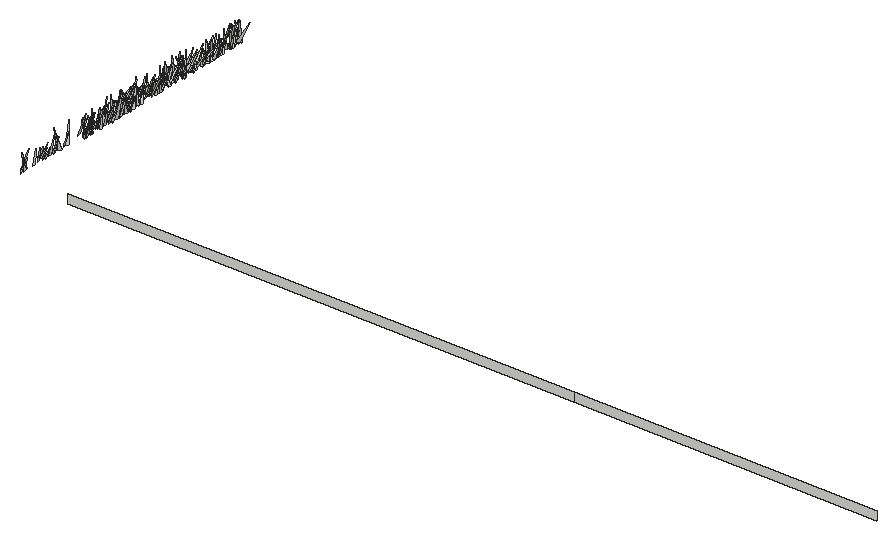
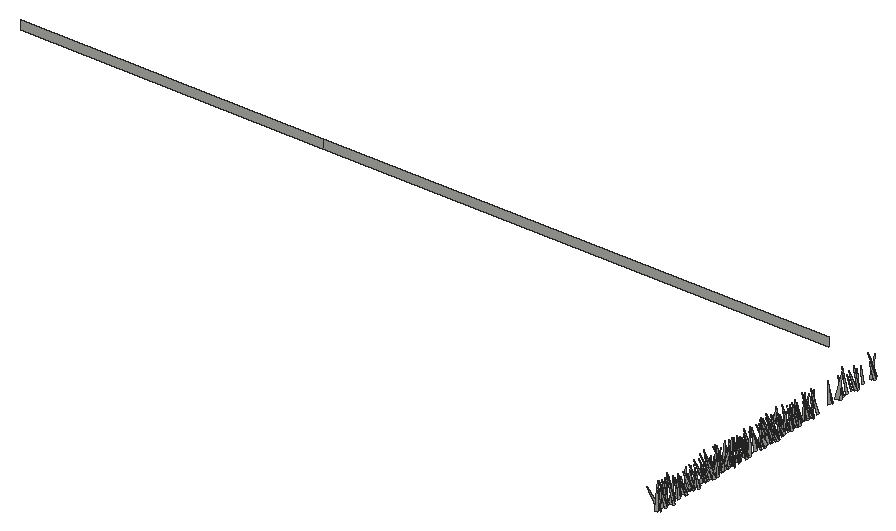
# SketchUp Ruby script. Lengths in inches.
U = 1.inch
M = Sketchup.active_model
def pt(a) = Geom::Point3d.new(a.map { |v| v * U })
def face(e, loops, mat)
  f = e.add_face(loops[0].map { |a| pt(a) })
  loops[1..].each { |l| e.add_face(l.map { |a| pt(a) }).erase! }
  f.material = f.back_material = mat if mat
  f
end
# faces: each face lists its corners as indices into pts; further lists are holes
def faces(e, pts, list, mat = nil) = list.each { |f| face(e, (f[0].is_a?(Array) ? f : [f]).map { |l| l.map { |i| pts[i] } }, mat) }
# xy, xz, yz: faces in a plane at the given z, y or x. An outline is a flat list of corners, or four numbers for a rectangle; further outlines are holes
def ring(l) = l.size == 4 ? [[l[0], l[1]], [l[2], l[1]], [l[2], l[3]], [l[0], l[3]]] : l.each_slice(2).to_a
def flat(e, list, mat, &to3) = list.each { |f| face(e, (f[0].is_a?(Array) ? f : [f]).map { |l| ring(l).map { |u, v| to3.(u, v) } }, mat) }
def xy(e, z, list, mat = nil) = flat(e, list, mat) { |x, y| [x, y, z] }
def xz(e, y, list, mat = nil) = flat(e, list, mat) { |x, z| [x, y, z] }
def yz(e, x, list, mat = nil) = flat(e, list, mat) { |y, z| [x, y, z] }
def lines(e, pts, list) = list.each { |a, b| e.add_line(pt(pts[a]), pt(pts[b])) }
# prism: a flat outline (further loops are holes) pulled along v
def prism(e, loops, v, mat = nil)
  f = face(e, loops, mat); d = Geom::Vector3d.new(v.map { |x| x * U })
  f.pushpull(f.normal.samedirection?(d) ? d.length : -d.length)
end
def box(e, o, s, mat = nil) = prism(e, [[o, [o[0] + s[0], o[1], o[2]], [o[0] + s[0], o[1] + s[1], o[2]], [o[0], o[1] + s[1], o[2]]]], [0, 0, s[2]], mat)
def at(x, y, z, deg = 0) = Geom::Transformation.translation(pt([x, y, z])) * Geom::Transformation.rotation(ORIGIN, Z_AXIS, deg.degrees)
def axes(o, x, y, z) = Geom::Transformation.new([*x, 0, *y, 0, *z, 0, *pt(o).to_a, 1])
def part(name) = M.definitions.add(name)
# library, detail: a bought-in or finely detailed component or shape, given as its bounding box
def library(name, o, s) = part(name).tap { |d| box(d.entities, o, s) }
def detail(e, o, s) = box(e.add_group.entities, o, s)
def put(e, d, t, mat = nil) = e.add_instance(d, t).tap { |i| i.material = mat if mat }
def group(e, t, mat = nil) = e.add_group.tap { |g| g.transformation = t; g.material = mat if mat }.entities
root = M.entities
c1 = part("fur_instance\#9")
p = [[0.8125,0,1.79],[0.67,-0.02,1.48],[0,-0.11,0],[0,0.11,0]]
faces(c1.entities,p,[[0,1,2,3]])
xz(root,5.77,[[196.6875,-27.625,525.63,-21.625],[525.63,-27.625,722.32,-21.625]])
put(root,c1,axes([157.51,131.72,-27.1],[2.91311,4.64162,1.0633],[4.76072,-2.81168,-0.76908],[0.10392,-1.30816,5.4258]))
put(root,c1,axes([159.54,140.72,-28.22],[-2.17535,-3.01047,0.60266],[-3.06621,2.16789,-0.23847],[0.15643,0.62897,3.70651]))
put(root,c1,axes([157.26,67.54,-28.22],[4.29125,3.34973,1.68987],[3.74545,-3.97458,-1.63261],[-0.21889,-2.33948,5.19327]))
put(root,c1,axes([160.47,87.49,-28.22],[-7.01031,-0.43579,1.43561],[-0.72042,6.99511,-1.39453],[1.31601,1.50792,6.88401]))
put(root,c1,axes([158.58,119.34,-28.22],[3.7026,-0.58317,1.91769],[-1.4169,-3.61072,1.63767],[-1.41775,2.08554,3.37155]))
put(root,c1,axes([156.99,160.79,-28.22],[0.56131,-6.10589,2.64479],[-6.41112,0.21442,1.85565],[1.78167,2.69518,5.8441]))
put(root,c1,axes([157.16,88.07,-27.1],[4.10425,1.09153,0.3293],[1.14011,-3.92312,-1.20584],[0.00571,-1.24998,4.07214]))
put(root,c1,axes([157.71,140.53,-27.1],[-1.05079,-7.8114,1.55453],[-7.7743,1.34665,1.51176],[1.73053,1.30661,7.73542]))
put(root,c1,axes([160.65,168.01,-28.22],[-4.27711,1.68369,0.0136],[1.68167,4.26988,0.26227],[-0.08344,-0.24902,4.58909]))
put(root,c1,axes([159.34,137.68,-28.22],[-4.78026,1.17069,2.19317],[1.89155,4.79719,1.56216],[1.61324,-2.15588,4.66702]))
put(root,c1,axes([156.68,18.28,-27.1],[2.75762,-4.13306,0.47465],[-3.98702,-2.46295,1.71739],[1.18791,1.32801,4.66232]))
put(root,c1,axes([156.68,188.21,-27.1],[2.75762,-4.13306,0.47465],[-3.98702,-2.46295,1.71739],[1.18791,1.32801,4.66232]))
put(root,c1,axes([158.6,80.15,-28.22],[-2.21972,3.26489,1.22418],[3.2229,2.47495,-0.75684],[1.3308,-0.54808,3.87477]))
put(root,c1,axes([159.18,164.24,-28.22],[-4.17455,0.44699,1.70239],[0.80041,4.38471,0.81146],[1.56757,-1.04848,4.11925]))
put(root,c1,axes([158.22,175.8125,-28.22],[4.13906,-0.88394,1.08396],[-0.87234,-4.27812,-0.15771],[-1.09332,0.06702,4.22946]))
put(root,c1,axes([159.26,127.18,-28.22],[6.19428,-1.57461,3.33029],[-1.87234,-6.95675,0.19327],[-3.17247,1.03131,6.38836]))
put(root,c1,axes([159.34,169.26,-28.22],[3.93388,5.26717,1.14139],[4.90502,-4.08461,1.94372],[-2.23307,0.30691,6.28017]))
put(root,c1,axes([157.5,170.05,-28.22],[4.34496,-0.35551,0.43941],[-0.4633,-4.19131,1.19014],[-0.32376,1.22666,4.19388]))
put(root,c1,axes([156.92,131.9,-28.22],[6.72288,3.05704,0.61475],[3.02645,-6.7488,0.46346],[-0.75102,0.16938,7.37074]))
put(root,c1,axes([157.94,132.77,-27.1],[-1.4348,-7.0433,2.45033],[-7.23254,1.92235,1.29061],[1.81726,2.08982,7.07114]))
put(root,c1,axes([159.1875,81.03,-28.22],[5.31201,5.41879,2.20999],[5.24419,-5.73235,1.45032],[-2.59727,-0.49162,7.44831]))
put(root,c1,axes([158.99,52.21,-27.1],[5.64429,-3.09602,3.33103],[-3.78051,-6.14532,0.69416],[-2.52761,2.27789,6.40012]))
put(root,c1,axes([159.05,102.86,-28.22],[2.70237,-4.42657,2.31196],[-4.83243,-2.98105,-0.05917],[-1.25989,1.93941,5.18593]))
put(root,c1,axes([158.375,149.63,-27.1],[-2.24137,-6.8028,0.2078],[-6.58087,2.22202,1.76064],[1.73594,-0.35988,6.94277]))
put(root,c1,axes([157.875,84.56,-28.22],[5.31281,-2.73186,1.51927],[-2.91837,-5.40827,0.48055],[-1.11999,1.13346,5.95467]))
put(root,c1,axes([160.2,108.16,-28.22],[-0.94907,-6.99906,3.73248],[-7.88487,0.42284,-1.21201],[-0.8643,3.82797,6.95835]))
put(root,c1,axes([157.1,33.07,-27.1],[5.55155,-0.72144,0.45458],[-0.77671,-5.51397,0.73462],[-0.35191,0.78896,5.54982]))
put(root,c1,axes([158.86,147.7,-28.22],[4.52461,-6.7861,0.00105],[-6.53347,-4.35651,-2.20405],[-1.83437,-1.22185,7.85273]))
put(root,c1,axes([158.53,76.12,-27.1],[0.17579,4.7582,1.26729],[4.89735,-0.03702,-0.54033],[0.51227,-1.27889,4.73069]))
put(root,c1,axes([156.77,181.63,-28.22],[-0.81294,-7.33898,4.00432],[-7.82592,2.08335,2.22952],[2.94113,3.51498,7.03923]))
put(root,c1,axes([158.62,108.45,-27.1],[3.88995,3.95886,0.07672],[3.75671,-3.72392,1.68217],[-1.25122,1.12695,5.2891]))
put(root,c1,axes([160.78,101.25,-28.22],[-1.75901,-6.72397,0.92553],[-6.70142,1.56883,-1.33876],[-1.07676,1.22044,6.82009]))
put(root,c1,axes([158.23,118.83,-28.22],[6.94101,-3.43299,1.84422],[-3.2352,-7.17632,-1.18245],[-2.17258,-0.28153,7.65277]))
put(root,c1,axes([159.31,89.31,-28.22],[-2.09366,4.25191,0.8072],[4.26644,2.17826,-0.40798],[0.72654,-0.53866,4.72184]))
put(root,c1,axes([157.43,45.27,-27.1],[2.80299,-5.03768,0.10257],[-5.00094,-2.76705,0.76127],[0.6159,0.45904,5.71449]))
put(root,c1,axes([160.36,93.08,-28.22],[-2.25031,-4.2676,0.76277],[-4.32128,2.13921,-0.77999],[-0.34742,1.03417,4.76108]))
put(root,c1,axes([158.22,143.05,-27.1],[-5.21121,-4.35385,3.58957],[-4.50193,6.15376,0.92827],[3.40202,1.4741,6.72689]))
put(root,c1,axes([160.66,133.85,-28.22],[-4.51725,1.3418,0.80765],[1.52463,4.33149,1.33117],[0.35811,-1.51528,4.52039]))
put(root,c1,axes([160.09,91.41,-28.22],[0.93593,4.40998,1.37185],[4.37962,-1.29175,1.16453],[-1.46587,-1.0437,4.3552]))
put(root,c1,axes([158.34,190.83,-28.22],[-3.30417,-4.76212,3.2823],[-5.25525,4.05058,0.5865],[2.41528,2.29867,5.7664]))
put(root,c1,axes([156.31,97,-27.1],[3.48936,7.09192,0.65775],[6.9322,-3.21357,-2.12629],[1.63479,-1.51038,7.61247]))
put(root,c1,axes([156.77,99.2,-27.1],[3.72746,5.46093,0.78491],[5.42353,-3.45332,-1.72965],[1.01153,-1.60767,6.38153]))
put(root,c1,axes([159.01,46.18,-27.1],[4.03591,-7.21522,0.98619],[-7.10178,-4.1491,-1.2924],[-1.61145,0.21471,8.16564]))
put(root,c1,axes([156.96,64.22,-27.1],[7.02887,1.41814,0.69885],[1.44367,-7.05544,-0.2028],[-0.64447,-0.3379,7.16763]))
put(root,c1,axes([156.72,97.48,-28.22],[6.03076,-3.95506,0.64167],[-4.00583,-5.92637,1.12057],[0.08689,1.28836,7.12438]))
put(root,c1,axes([158.94,18.03,-27.1],[5.89812,-2.41371,1.85981],[-1.99813,-6.12286,-1.60962],[-2.30052,-0.87028,6.16628]))
put(root,c1,axes([158.94,187.96,-27.1],[5.89812,-2.41371,1.85981],[-1.99813,-6.12286,-1.60962],[-2.30052,-0.87028,6.16628]))
put(root,c1,axes([160.3,144.44,-28.22],[-3.47143,-2.84551,0.09651],[-2.81271,3.45107,0.57956],[0.4415,-0.38766,4.45106]))
put(root,c1,axes([160.62,66.03,-28.22],[-3.27995,-3.84872,1.10692],[-4.00472,3.15616,-0.89264],[0.01123,1.42196,4.97734]))
put(root,c1,axes([159.04,133.15,-27.1],[-0.27729,4.76979,1.49646],[4.98187,0.38774,-0.31274],[0.41383,-1.47171,4.7676]))
put(root,c1,axes([160.15,145.42,-28.22],[-5.81537,-0.03657,1.70774],[-0.23888,6.01751,-0.6846],[1.69135,0.72416,5.77505]))
put(root,c1,axes([158.2,127.17,-28.22],[4.35259,2.65064,0.87547],[2.69973,-4.40951,-0.0717],[-0.70982,-0.51745,5.09567]))
put(root,c1,axes([159.85,106.57,-28.22],[1.43677,3.63281,1.03111],[3.57622,-1.66329,0.8769],[-1.21291,-0.60083,3.80693]))
put(root,c1,axes([158.41,120.52,-27.1],[2.85218,4.71528,1.10181],[4.83661,-2.83604,-0.38317],[-0.23454,-1.14272,5.49745]))
put(root,c1,axes([159.67,152.3,-28.22],[1.56672,2.93333,1.48069],[3.11219,-1.85095,0.37383],[-1.05412,-1.105,3.30444]))
put(root,c1,axes([158.59,152.92,-28.22],[4.55494,-1.38322,1.77977],[-1.90749,-4.50337,1.38185],[-1.20098,1.9065,4.55536]))
put(root,c1,axes([159.9,164.69,-28.22],[-3.4412,6.39637,0.09759],[6.32165,3.41718,-1.06042],[0.97968,0.41743,7.18546]))
put(root,c1,axes([159.03,92.17,-27.1],[-2.22453,-2.28888,1.93607],[-2.6411,2.63697,0.08289],[1.41842,1.32035,3.19071]))
put(root,c1,axes([158.59,100.56,-27.1],[-1.16046,8.00046,0.20395],[7.87345,1.17823,-1.41992],[1.43448,0.00519,7.95851]))
put(root,c1,axes([158.07,30.12,-27.1],[4.83385,-1.43847,0.54232],[-1.36908,-4.84202,-0.64023],[-0.69925,-0.46374,5.00254]))
put(root,c1,axes([158.26,125.71,-28.22],[4.95919,2.18923,1.00137],[2.21006,-5.04934,0.09393],[-0.95452,-0.31696,5.4201]))
put(root,c1,axes([158.61,19.19,-27.1],[4.29129,-1.7599,0.57931],[-1.53313,-4.1935,-1.38278],[-1.04037,-1.07949,4.42723]))
put(root,c1,axes([158.61,189.125,-27.1],[4.29129,-1.7599,0.57931],[-1.53313,-4.1935,-1.38278],[-1.04037,-1.07949,4.42723]))
put(root,c1,axes([160.19,154.14,-28.22],[2.70067,-3.13661,0.88183],[-2.51329,-2.73437,-2.02883],[-2.07348,-0.77102,3.60774]))
put(root,c1,axes([158.07,100.87,-28.22],[5.62974,5.25868,1.12192],[5.27805,-5.71471,0.30107],[-1.02693,-0.54292,7.69786]))
put(root,c1,axes([158.71,70.54,-27.1],[3.49135,-1.63355,1.08284],[-1.80913,-3.53699,0.49727],[-0.7537,0.9229,3.8224]))
put(root,c1,axes([158.75,133.85,-28.22],[-0.66532,-4.77379,0.4836],[-4.67341,0.75535,1.0268],[1.0873,0.32553,4.70929]))
put(root,c1,axes([156.36,111.21,-27.1],[1.31269,5.55847,0.82299],[4.82858,-0.68361,-3.08457],[2.8738,-1.39037,4.80678]))
put(root,c1,axes([157.73,67.33,-28.22],[-0.77489,5.32124,0.74593],[4.8544,1.01638,-2.20776],[2.30365,-0.35187,4.90325]))
put(root,c1,axes([158.58,77.17,-28.22],[6.13024,0.22864,1.74835],[0.20896,-6.37456,0.10097],[-1.75081,0.03976,6.13367]))
put(root,c1,axes([159.04,112.39,-28.22],[-5.57842,3.33095,2.99608],[3.28064,6.29556,-0.89096],[3.05108,-0.67911,6.43585]))
put(root,c1,axes([158.82,181.64,-28.22],[6.05759,-4.04132,1.47541],[-3.82561,-6.22554,-1.34569],[-1.96821,-0.33746,7.15653]))
put(root,c1,axes([158.15,126.125,-28.22],[5.73568,-0.06882,1.05766],[0.01363,-5.81521,-0.45231],[-1.05981,-0.44725,5.71823]))
put(root,c1,axes([156.54,31.98,-27.1],[0.60809,-6.43634,0.77652],[-5.71222,-0.16309,3.1214],[3.06594,0.97271,5.66154]))
put(root,c1,axes([157.8,132.78,-27.1],[7.1612,-0.61813,1.17268],[-0.1707,-6.81898,-2.55193],[-1.31459,-2.48182,6.71956]))
put(root,c1,axes([159.02,25.45,-27.1],[4.44334,-1.86269,1.64457],[-2.02269,-4.66849,0.17731],[-1.44323,0.80817,4.81471]))
put(root,c1,axes([159.34,77.1,-28.22],[3.35457,-1.66316,1.27005],[-1.64462,-3.57909,-0.343],[-1.29397,0.23728,3.72849]))
put(root,c1,axes([159.68,105.95,-28.22],[-2.87037,3.7349,1.34525],[3.80013,3.06525,-0.40189],[1.14815,-0.80807,4.69329]))
put(root,c1,axes([159.9,190.56,-28.22],[-6.01027,1.97565,2.91231],[2.62602,6.35479,1.10849],[2.3428,-2.05464,6.22879]))
put(root,c1,axes([160.58,145.71,-28.22],[0.5538,7.06628,1.29605],[7.05626,-0.7792,1.23321],[-1.34954,-1.17443,6.97985]))
put(root,c1,axes([160.18,175.52,-28.22],[-4.8782,2.33838,1.88669],[2.5546,5.12175,0.25721],[1.58166,-1.06025,5.40358]))
put(root,c1,axes([157.15,148.13,-28.22],[4.70932,-5.02611,1.74089],[-5.27526,-4.11549,2.38842],[0.68127,2.87596,6.46026]))
put(root,c1,axes([158.18,132.29,-27.1],[-3.37811,-5.89928,1.5704],[-5.1932,3.72048,2.80499],[3.2091,-0.18922,6.19235]))
put(root,c1,axes([157.73,121.45,-27.1],[5.98567,0.36805,0.66862],[0.55714,-5.71998,-1.83907],[-0.52163,-1.88604,5.70802]))
put(root,c1,axes([159.59,163.13,-28.22],[3.73887,4.62596,1.90486],[4.75099,-4.02818,0.45718],[-1.5672,-1.17533,5.9304]))
put(root,c1,axes([158.62,153.15,-28.22],[-0.57371,3.97778,1.97621],[4.19128,1.14438,-1.08668],[1.47014,-1.71025,3.86924]))
put(root,c1,axes([159.96,160.79,-28.22],[1.30026,-4.12004,1.09762],[-4.18224,-1.45572,-0.50983],[-0.82967,0.8811,4.29016]))
put(root,c1,axes([158.39,91.97,-28.22],[-3.91032,-4.73518,3.93684],[-5.20514,5.03349,0.88414],[3.29046,2.33522,6.07707]))
put(root,c1,axes([158.91,32.74,-27.1],[3.66327,1.41122,0.72087],[1.44956,-3.71776,-0.08822],[-0.64027,-0.34277,3.92471]))
put(root,c1,axes([158.33,75.24,-27.1],[1.81296,4.05322,0.9149],[4.0683,-1.5284,-1.29051],[0.84535,-1.3371,4.24853]))
put(root,c1,axes([159.4,140.83,-28.22],[5.90361,-0.69248,2.28384],[-0.937,-6.27702,0.51884],[-2.19488,0.81708,5.9214]))
put(root,c1,axes([160.61,101.7,-28.22],[-0.82643,-5.48525,0.94931],[-5.54864,0.73423,-0.58792],[-0.44918,1.02229,5.51591]))
put(root,c1,axes([157.02,106.21,-27.1],[5.8068,-2.41673,0.19711],[-2.36119,-5.5195,1.88633],[0.55156,1.81463,6.0001]))
put(root,c1,axes([157.46,145.39,-28.22],[6.93671,-0.62868,0.23505],[-0.51232,-6.5363,-2.3628],[-0.4336,-2.33453,6.55213]))
put(root,c1,axes([160.07,165.4,-28.22],[-2.64442,5.36733,3.49605],[6.32318,2.79183,0.49668],[1.02376,-3.3795,5.96276]))
put(root,c1,axes([157.11,121.88,-28.22],[1.83372,-5.8574,1.52699],[-5.60076,-1.03656,2.74963],[2.29617,2.14936,5.48737]))
put(root,c1,axes([158.85,93.19,-27.1],[0.22976,-4.49295,1.68417],[-4.67204,0.17468,1.10336],[1.09322,1.69077,4.36142]))
put(root,c1,axes([160.43,153.19,-28.22],[-4.5247,0.14497,1.56827],[-0.47946,4.4174,-1.79167],[1.5002,1.84904,4.15738]))
put(root,c1,axes([158.49,66.45,-28.22],[6.71372,1.26121,1.18447],[0.98901,-6.69183,1.51954],[-1.41968,1.3025,6.66001]))
put(root,c1,axes([159.29,81.3,-28.22],[-3.8078,3.44308,3.43375],[4.19662,4.52997,0.11149],[2.45637,-2.40193,5.13242]))
put(root,c1,axes([157.74,106.58,-28.22],[3.29636,-5.4576,1.30622],[-5.51274,-2.86598,1.93739],[1.04942,2.08768,6.07437]))
put(root,c1,axes([159.21,71.92,-28.22],[6.08028,3.66314,2.96745],[4.34842,-6.22849,-1.22118],[-1.82087,-2.64225,6.99265]))
put(root,c1,axes([159.91,128.46,-28.22],[1.54833,5.59255,0.52827],[5.59137,-1.58705,0.41342],[-0.54067,-0.39706,5.78818]))
put(root,c1,axes([157.85,132.48,-27.1],[6.64533,-1.36705,0.39109],[-1.31179,-6.61549,-0.83466],[-0.54862,-0.74069,6.73295]))
put(root,c1,axes([160.1,104.91,-28.22],[-3.98978,2.11987,2.03955],[2.3526,4.36264,0.06771],[1.76604,-1.02247,4.51748]))
put(root,c1,axes([158.6,14.89,-27.1],[5.3088,5.05785,1.00754],[5.10033,-5.36326,0.04959],[-0.76398,-0.65873,7.33231]))
put(root,c1,axes([158.6,184.82,-27.1],[5.3088,5.05785,1.00754],[5.10033,-5.36326,0.04959],[-0.76398,-0.65873,7.33231]))
put(root,c1,axes([158.65,134.3125,-27.1],[3.34726,-4.07819,1.53745],[-4.35777,-3.09938,1.26621],[0.07255,1.99042,5.12177]))
put(root,c1,axes([157.65,68.67,-27.1],[5.84375,1.80801,0.13219],[1.81029,-5.79638,-0.74876],[0.09603,-0.75425,6.07105]))
put(root,c1,axes([159.68,173.51,-28.22],[0.13174,-4.85064,1.64659],[-5.10405,0.01535,0.4536],[0.43432,1.65178,4.83118]))
put(root,c1,axes([160.75,110.71,-28.22],[-3.45785,1.40655,0.59459],[1.25916,3.45892,-0.85969],[0.86397,0.58836,3.63264]))
put(root,c1,axes([157.58,78.17,-28.22],[2.64878,-6.42579,1.07864],[-6.29914,-2.22772,2.19734],[1.66585,1.79353,6.59382]))
put(root,c1,axes([158.59,78.36,-28.22],[6.30339,2.19635,1.13005],[2.22882,-6.39265,-0.00763],[-1.06457,-0.37914,6.67507]))
put(root,c1,axes([157.79,179.88,-28.22],[7.78659,2.72532,1.24866],[2.87625,-7.77148,-0.97412],[-0.84485,-1.33952,8.19204]))
put(root,c1,axes([158.1,100.26,-28.22],[3.64323,6.95762,0.66244],[6.95502,-3.53547,-1.11744],[0.68929,-1.10109,7.77386]))
put(root,c1,axes([158.26,50.41,-27.1],[4.88732,1.92922,0.49219],[1.99044,-4.76555,-1.08522],[-0.04774,-1.19066,5.14102]))
put(root,c1,axes([160.37,98.42,-28.22],[-0.06677,3.94377,1.582],[4.24655,0.00562,0.16522],[-0.15123,-1.5834,3.94087]))
put(root,c1,axes([159,72.26,-27.1],[3.9114,-1.46291,0.01114],[-1.40736,-3.77134,-1.11157],[-0.39945,-1.03737,4.02536]))
put(root,c1,axes([158.96,73.99,-27.1],[5.13341,-1.95182,0.40555],[-1.78394,-4.9977,-1.47188],[-0.88973,-1.24068,5.29103]))
put(root,c1,axes([160.34,166.39,-28.22],[-1.20745,-5.31811,1.49773],[-5.50418,1.29079,0.14593],[0.47907,1.42653,5.45151]))
put(root,c1,axes([160.36,111,-28.22],[0.70725,4.81258,1.31899],[4.97344,-0.78845,0.21001],[-0.40688,-1.27212,4.85974]))
put(root,c1,axes([158.33,41.91,-27.1],[3.55889,4.26793,1.49162],[4.48448,-3.09137,-1.85436],[0.57409,-2.30955,5.23854]))
put(root,c1,axes([158.25,89.77,-28.22],[6.37696,0.70596,0.43543],[0.57496,-6.19552,1.62437],[-0.59783,1.57187,6.20688]))
put(root,c1,axes([159.21,183.1,-28.22],[6.67173,1.075,1.66778],[0.88806,-6.84957,0.86244],[-1.77439,0.61387,6.70252]))
put(root,c1,axes([160.64,176.85,-28.22],[-1.59242,3.59476,0.56652],[3.61736,1.63113,-0.18207],[0.39739,-0.44291,3.92746]))
put(root,c1,axes([158.81,122.24,-27.1],[4.67229,-0.63233,0.28263],[-0.57173,-4.60903,-0.86025],[-0.39095,-0.81674,4.63574]))
put(root,c1,axes([158,151,-27.1],[2.12208,6.92928,3.4126],[7.54208,-1.09525,-2.46604],[1.66665,-3.86645,6.81445]))
put(root,c1,axes([159.875,105.93,-28.22],[2.54214,-2.62214,0.84113],[-2.70032,-2.59808,0.06187],[-0.53981,0.64801,3.65161]))
put(root,c1,axes([158.7,135.62,-28.22],[0.07577,6.70614,0.84141],[6.48392,0.16538,-1.90197],[1.90764,-0.82847,6.43122]))
put(root,c1,axes([159.875,175.8,-28.22],[-3.52584,-3.38703,1.52089],[-2.9555,3.82986,1.67745],[2.24724,-0.27722,4.59235]))
put(root,c1,axes([159.08,169.38,-28.22],[7.02659,-0.33713,1.59],[0.09653,-6.95626,-1.90152],[-1.62247,-1.87389,6.7728]))
put(root,c1,axes([160.23,155.35,-28.22],[1.07632,-4.38935,0.89904],[-4.4763,-1.09335,0.02097],[-0.19334,0.87825,4.51934]))
put(root,c1,axes([158.59,38.66,-27.1],[6.87118,-2.4682,1.14103],[-2.53265,-6.93781,0.24398],[-0.98977,0.61792,7.29696]))
put(root,c1,axes([160.36,64.59,-28.22],[-3.10043,-5.65859,2.0595],[-5.81568,3.41455,0.62657],[1.56175,1.48157,6.42182]))
put(root,c1,axes([159.22,183.76,-28.22],[2.91311,4.64162,1.0633],[4.76072,-2.81168,-0.76908],[0.10392,-1.30816,5.4258]))
put(root,c1,axes([157.54,87.45,-27.1],[1.03631,-6.95808,1.71035],[-6.57848,-0.23906,3.0134],[2.83968,1.98547,6.35675]))
put(root,c1,axes([158.81,117.71,-27.1],[3.25053,-3.28963,0.28157],[-3.26975,-3.15258,0.91484],[0.45796,0.84053,4.53329]))
put(root,c1,axes([158.87,140.11,-28.22],[4.10425,1.09153,0.3293],[1.14011,-3.92312,-1.20584],[0.00571,-1.24998,4.07214]))
put(root,c1,axes([159.42,192.57,-28.22],[-1.05079,-7.8114,1.55453],[-7.7743,1.34665,1.51176],[1.73053,1.30661,7.73542]))
put(root,c1,axes([158.73,42.04,-27.1],[5.12871,-2.48578,0.55768],[-2.53054,-5.11559,0.47007],[-0.29413,0.66743,5.67995]))
put(root,c1,axes([158.39,70.32,-28.22],[2.75762,-4.13306,0.47465],[-3.98702,-2.46295,1.71739],[1.18791,1.32801,4.66232]))
put(root,c1,axes([157.79,138.14,-27.1],[6.83257,-2.01041,0.78824],[-2.1593,-6.33413,2.56189],[0.022,2.68032,6.64549]))
put(root,c1,axes([159.65,184.81,-28.22],[-1.4348,-7.0433,2.45033],[-7.23254,1.92235,1.29061],[1.81726,2.08982,7.07114]))
put(root,c1,axes([160.7,104.25,-28.22],[5.64429,-3.09602,3.33103],[-3.78051,-6.14532,0.69416],[-2.52761,2.27789,6.40012]))
put(root,c1,axes([158.8125,85.11,-28.22],[5.55155,-0.72144,0.45458],[-0.77671,-5.51397,0.73462],[-0.35191,0.78896,5.54982]))
put(root,c1,axes([160.24,128.16,-28.22],[0.17579,4.7582,1.26729],[4.89735,-0.03702,-0.54033],[0.51227,-1.27889,4.73069]))
put(root,c1,axes([160.33,160.49,-28.22],[3.88995,3.95886,0.07672],[3.75671,-3.72392,1.68217],[-1.25122,1.12695,5.2891]))
put(root,c1,axes([158.97,34.61,-27.1],[2.19638,-3.75423,0.49776],[-3.62923,-1.92217,1.51658],[1.08198,1.1735,4.07656]))
put(root,c1,axes([159.14,97.32,-28.22],[2.80299,-5.03768,0.10257],[-5.00094,-2.76705,0.76127],[0.6159,0.45904,5.71449]))
put(root,c1,axes([158.02,149.04,-28.22],[3.48936,7.09192,0.65775],[6.9322,-3.21357,-2.12629],[1.63479,-1.51038,7.61247]))
put(root,c1,axes([158.48,151.24,-28.22],[3.72746,5.46093,0.78491],[5.42353,-3.45332,-1.72965],[1.01153,-1.60767,6.38153]))
put(root,c1,axes([160.72,98.22,-28.22],[4.03591,-7.21522,0.98619],[-7.10178,-4.1491,-1.2924],[-1.61145,0.21471,8.16564]))
put(root,c1,axes([158.67,116.26,-28.22],[7.02887,1.41814,0.69885],[1.44367,-7.05544,-0.2028],[-0.64447,-0.3379,7.16763]))
put(root,c1,axes([160.66,70.08,-28.22],[5.89812,-2.41371,1.85981],[-1.99813,-6.12286,-1.60962],[-2.30052,-0.87028,6.16628]))
put(root,c1,axes([160.75,185.19,-28.22],[-0.27729,4.76979,1.49646],[4.98187,0.38774,-0.31274],[0.41383,-1.47171,4.7676]))
put(root,c1,axes([160.12,172.5625,-28.22],[2.85218,4.71528,1.10181],[4.83661,-2.83604,-0.38317],[-0.23454,-1.14272,5.49745]))
put(root,c1,axes([160.74,144.21,-28.22],[-2.22453,-2.28888,1.93607],[-2.6411,2.63697,0.08289],[1.41842,1.32035,3.19071]))
put(root,c1,axes([160.3,152.6,-28.22],[-1.16046,8.00046,0.20395],[7.87345,1.17823,-1.41992],[1.43448,0.00519,7.95851]))
put(root,c1,axes([159.78,82.16,-28.22],[4.83385,-1.43847,0.54232],[-1.36908,-4.84202,-0.64023],[-0.69925,-0.46374,5.00254]))
put(root,c1,axes([160.32,71.24,-28.22],[4.29129,-1.7599,0.57931],[-1.53313,-4.1935,-1.38278],[-1.04037,-1.07949,4.42723]))
put(root,c1,axes([160.42,122.58,-28.22],[3.49135,-1.63355,1.08284],[-1.80913,-3.53699,0.49727],[-0.7537,0.9229,3.8224]))
put(root,c1,axes([158.07,163.25,-28.22],[1.31269,5.55847,0.82299],[4.82858,-0.68361,-3.08457],[2.8738,-1.39037,4.80678]))
put(root,c1,axes([158.25,84.02,-28.22],[0.60809,-6.43634,0.77652],[-5.71222,-0.16309,3.1214],[3.06594,0.97271,5.66154]))
put(root,c1,axes([159.51,184.82,-28.22],[7.1612,-0.61813,1.17268],[-0.1707,-6.81898,-2.55193],[-1.31459,-2.48182,6.71956]))
put(root,c1,axes([160.73,77.49,-28.22],[4.44334,-1.86269,1.64457],[-2.02269,-4.66849,0.17731],[-1.44323,0.80817,4.81471]))
put(root,c1,axes([159.89,184.33,-28.22],[-3.37811,-5.89928,1.5704],[-5.1932,3.72048,2.80499],[3.2091,-0.18922,6.19235]))
put(root,c1,axes([159.4375,173.49,-28.22],[5.98567,0.36805,0.66862],[0.55714,-5.71998,-1.83907],[-0.52163,-1.88604,5.70802]))
put(root,c1,axes([160.62,84.78,-28.22],[3.66327,1.41122,0.72087],[1.44956,-3.71776,-0.08822],[-0.64027,-0.34277,3.92471]))
put(root,c1,axes([160.04,127.28,-28.22],[1.81296,4.05322,0.9149],[4.0683,-1.5284,-1.29051],[0.84535,-1.3371,4.24853]))
put(root,c1,axes([158.73,158.25,-28.22],[5.8068,-2.41673,0.19711],[-2.36119,-5.5195,1.88633],[0.55156,1.81463,6.0001]))
put(root,c1,axes([160.56,145.23,-28.22],[0.22976,-4.49295,1.68417],[-4.67204,0.17468,1.10336],[1.09322,1.69077,4.36142]))
put(root,c1,axes([159.5625,184.52,-28.22],[6.64533,-1.36705,0.39109],[-1.31179,-6.61549,-0.83466],[-0.54862,-0.74069,6.73295]))
put(root,c1,axes([160.31,66.93,-28.22],[5.3088,5.05785,1.00754],[5.10033,-5.36326,0.04959],[-0.76398,-0.65873,7.33231]))
put(root,c1,axes([160.36,186.35,-28.22],[3.34726,-4.07819,1.53745],[-4.35777,-3.09938,1.26621],[0.07255,1.99042,5.12177]))
put(root,c1,axes([159.36,120.71,-28.22],[5.84375,1.80801,0.13219],[1.81029,-5.79638,-0.74876],[0.09603,-0.75425,6.07105]))
put(root,c1,axes([159.97,102.45,-28.22],[4.88732,1.92922,0.49219],[1.99044,-4.76555,-1.08522],[-0.04774,-1.19066,5.14102]))
put(root,c1,axes([160.71,124.3,-28.22],[3.9114,-1.46291,0.01114],[-1.40736,-3.77134,-1.11157],[-0.39945,-1.03737,4.02536]))
put(root,c1,axes([160.67,126.04,-28.22],[5.13341,-1.95182,0.40555],[-1.78394,-4.9977,-1.47188],[-0.88973,-1.24068,5.29103]))
put(root,c1,axes([160.04,93.96,-28.22],[3.55889,4.26793,1.49162],[4.48448,-3.09137,-1.85436],[0.57409,-2.30955,5.23854]))
put(root,c1,axes([160.52,174.28,-28.22],[4.67229,-0.63233,0.28263],[-0.57173,-4.60903,-0.86025],[-0.39095,-0.81674,4.63574]))
put(root,c1,axes([160.3,90.7,-28.22],[6.87118,-2.4682,1.14103],[-2.53265,-6.93781,0.24398],[-0.98977,0.61792,7.29696]))
put(root,c1,axes([159.25,139.5,-28.22],[1.03631,-6.95808,1.71035],[-6.57848,-0.23906,3.0134],[2.83968,1.98547,6.35675]))
put(root,c1,axes([160.52,169.76,-28.22],[3.25053,-3.28963,0.28157],[-3.26975,-3.15258,0.91484],[0.45796,0.84053,4.53329]))
put(root,c1,axes([160.4375,94.08,-28.22],[5.12871,-2.48578,0.55768],[-2.53054,-5.11559,0.47007],[-0.29413,0.66743,5.67995]))
put(root,c1,axes([159.5,190.18,-28.22],[6.83257,-2.01041,0.78824],[-2.1593,-6.33413,2.56189],[0.022,2.68032,6.64549]))
put(root,c1,axes([160.68,86.66,-28.22],[2.19638,-3.75423,0.49776],[-3.62923,-1.92217,1.51658],[1.08198,1.1735,4.07656]))
